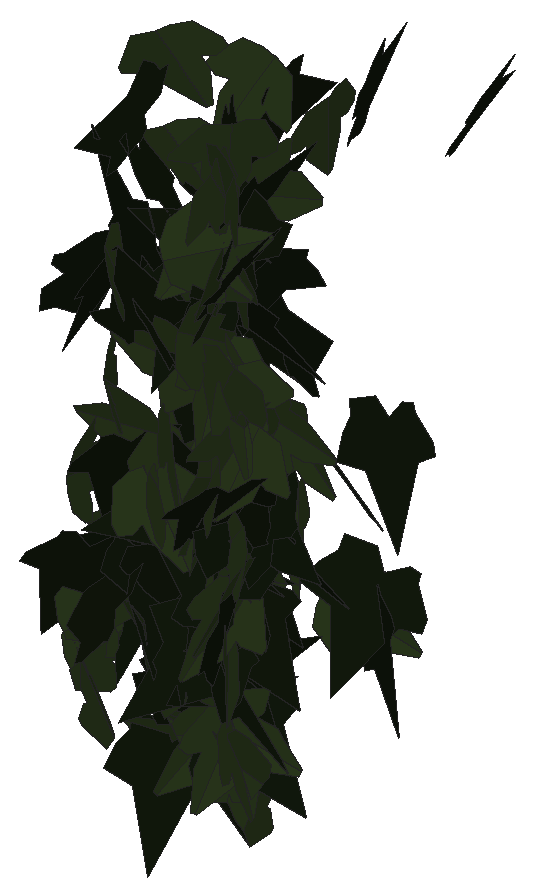
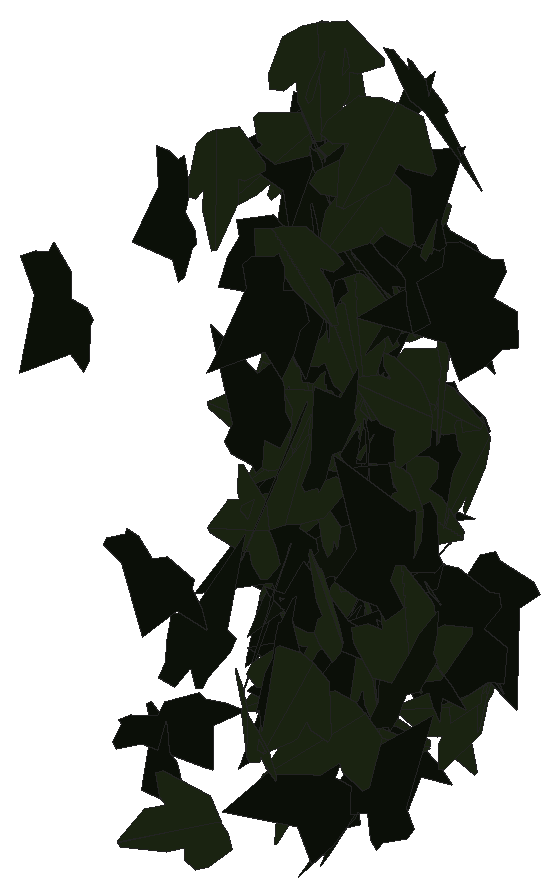
# SketchUp Ruby script. Lengths in inches.
U = 1.inch
M = Sketchup.active_model
def pt(a) = Geom::Point3d.new(a.map { |v| v * U })
def face(e, loops, mat)
  f = e.add_face(loops[0].map { |a| pt(a) })
  loops[1..].each { |l| e.add_face(l.map { |a| pt(a) }).erase! }
  f.material = f.back_material = mat if mat
  f
end
# faces: each face lists its corners as indices into pts; further lists are holes
def faces(e, pts, list, mat = nil) = list.each { |f| face(e, (f[0].is_a?(Array) ? f : [f]).map { |l| l.map { |i| pts[i] } }, mat) }
# xy, xz, yz: faces in a plane at the given z, y or x. An outline is a flat list of corners, or four numbers for a rectangle; further outlines are holes
def ring(l) = l.size == 4 ? [[l[0], l[1]], [l[2], l[1]], [l[2], l[3]], [l[0], l[3]]] : l.each_slice(2).to_a
def flat(e, list, mat, &to3) = list.each { |f| face(e, (f[0].is_a?(Array) ? f : [f]).map { |l| ring(l).map { |u, v| to3.(u, v) } }, mat) }
def xy(e, z, list, mat = nil) = flat(e, list, mat) { |x, y| [x, y, z] }
def xz(e, y, list, mat = nil) = flat(e, list, mat) { |x, z| [x, y, z] }
def yz(e, x, list, mat = nil) = flat(e, list, mat) { |y, z| [x, y, z] }
def lines(e, pts, list) = list.each { |a, b| e.add_line(pt(pts[a]), pt(pts[b])) }
# prism: a flat outline (further loops are holes) pulled along v
def prism(e, loops, v, mat = nil)
  f = face(e, loops, mat); d = Geom::Vector3d.new(v.map { |x| x * U })
  f.pushpull(f.normal.samedirection?(d) ? d.length : -d.length)
end
def box(e, o, s, mat = nil) = prism(e, [[o, [o[0] + s[0], o[1], o[2]], [o[0] + s[0], o[1] + s[1], o[2]], [o[0], o[1] + s[1], o[2]]]], [0, 0, s[2]], mat)
def at(x, y, z, deg = 0) = Geom::Transformation.translation(pt([x, y, z])) * Geom::Transformation.rotation(ORIGIN, Z_AXIS, deg.degrees)
def axes(o, x, y, z) = Geom::Transformation.new([*x, 0, *y, 0, *z, 0, *pt(o).to_a, 1])
def part(name) = M.definitions.add(name)
# library, detail: a bought-in or finely detailed component or shape, given as its bounding box
def library(name, o, s) = part(name).tap { |d| box(d.entities, o, s) }
def detail(e, o, s) = box(e.add_group.entities, o, s)
def put(e, d, t, mat = nil) = e.add_instance(d, t).tap { |i| i.material = mat if mat }
def group(e, t, mat = nil) = e.add_group.tap { |g| g.transformation = t; g.material = mat if mat }.entities
root = M.entities
M.materials.add("efeu1").color = [18, 25, 13]
M.materials.add("efeu2").color = [43, 57, 29]
c1 = part("ivyleaf_9")
p = [[1.54,2.16,1.25],[1.36,2.04,1.19],[-0.21,0.99,0.68],[-0.71,1.11,0.82],[-0.85,0.86,0.67],[-0.8,0.17,0.21],
  [-0.9,-0.01,0.1],[-0.67,-0.16,-0.02],[-0.08,-0.08,-0.05],[-0.03,-0.6,-0.4],[0.65,-0.88,-0.66],[0.83,-0.6,-0.49],
  [1.29,-0.42,-0.43],[1.8125,-0.07,-0.26],[1.21,0.44,0.15]]
faces(c1.entities,p,[[0,1,2,3,4,5,6,7,8,9,10,11,12,13,14]],"efeu1")
c2 = part("ivyleaf_10")
p = [[0,0.5,-0.03],[-0.0625,2.02,-0.43],[-0.19,2.01,-0.46],[-0.54,1.05,-0.29],[-0.52,0.625,-0.18],[-0.83,0.76,-0.28],
  [-1.16,0.64,-0.33],[-1.15,0.33,-0.24],[-0.77,-0.39,0.02],[-0.3,-0.51,0.16],[0.04,-0.48,0.23],[-0.02,2.01,-0.4375],
  [-0.06,2.01,-0.43],[0.04,-0.49,0.23],[0.67,-0.49,0.14],[1.38,0.36,-0.2],[1.375,0.51,-0.24],[0.81,0.65,-0.19],
  [0.62,0.59,-0.15],[0.6,1.09,-0.28],[0.5,1.23,-0.31]]
faces(c2.entities,p,[[0,1,2,3,4,5,6,7,8,9,10],[11,12,0,13,14,15,16,17,18,19,20]],"efeu2")
put(root,c1,axes([43.95,223.39,216.41],[0.08956,-0.30922,0.38258],[0.18004,-0.34128,-0.31799],[0.45778,0.19471,0.05022]))
put(root,c2,axes([44.24,222.97,216.52],[-0.36083,-0.34597,0.01044],[0.01621,-0.00184,0.49973],[-0.34575,0.36097,0.01254]))
put(root,c1,axes([44.42,221.74,216.83],[0.11394,0.33343,-0.35474],[-0.11745,-0.33474,-0.35236],[-0.47246,0.16363,0.00204]))
put(root,c2,axes([44.09,224.26,216.3125],[-0.31231,-0.10129,-0.3771],[0.37075,0.07456,-0.32708],[0.12249,-0.48392,0.02854]))
put(root,c2,axes([44.33,224.72,216.98],[-0.46824,0.06808,-0.16162],[0.15837,-0.03375,-0.47305],[-0.07532,-0.49419,0.01004]))
put(root,c1,axes([44.22,221.66,220.34],[0.04575,0.29571,-0.40057],[0.03546,0.39931,0.29883],[0.49664,-0.05575,0.01557]))
put(root,c2,axes([44.29,221.84,215.41],[0.05774,0.1204,-0.48184],[0.22281,0.42725,0.13346],[0.44387,-0.23013,-0.00431]))
put(root,c2,axes([44.25,221.83,215.86],[0.09592,0.11629,-0.47674],[0.3131,0.35952,0.15069],[0.37784,-0.32745,-0.00385]))
put(root,c1,axes([44.11,221.94,216.47],[0.16385,0.18519,-0.43458],[0.29229,0.3216,0.24726],[0.3711,-0.33508,-0.00287]))
put(root,c1,axes([44.53,222.65,216.38],[-0.41427,-0.07728,-0.26909],[0.2623,0.06092,-0.4213],[0.0979,-0.49022,-0.00993]))
put(root,c2,axes([44.68,221.26,218.1],[-0.03233,0.14031,0.47882],[-0.24713,0.41233,-0.13751],[-0.43345,-0.24556,0.04269]))
put(root,c1,axes([44.72,223.02,214.55],[0.21831,-0.23563,0.38317],[-0.26691,0.27497,0.32117],[-0.36207,-0.34478,-0.00573]))
put(root,c2,axes([44.83,221.46,214.94],[-0.25641,0.20819,-0.37538],[-0.28386,0.24576,0.33019],[0.322,0.38244,-0.00784]))
put(root,c2,axes([44.24,222.9,219.52],[-0.06761,0.04814,-0.49306],[0.4406,-0.22166,-0.08206],[-0.22649,-0.44559,-0.01244]))
put(root,c1,axes([44.78,221.84,220.7],[-0.21326,0.35811,-0.27618],[0.13344,-0.24192,-0.41673],[-0.4321,-0.25145,0.00761]))
put(root,c2,axes([44.59,223.84,217.18],[0.30463,-0.39277,0.05415],[-0.02943,0.0457,0.49704],[-0.39539,-0.30601,0.00472]))
put(root,c2,axes([44.61,222.92,222.875],[-0.40226,-0.22618,-0.19243],[0.16184,0.10468,-0.46136],[0.24899,-0.43346,-0.011]))
put(root,c1,axes([45.02,221.42,216.43],[-0.28644,0.35543,0.20401],[-0.1375,0.15113,-0.45635],[-0.38607,-0.31754,0.01116]))
put(root,c1,axes([44.49,222.68,217.41],[0.22441,0.43966,0.07963],[-0.04676,-0.06551,0.49348],[0.44436,-0.22893,0.01172]))
put(root,c2,axes([44.81,224.32,221.95],[0.45297,-0.0278,-0.20986],[-0.20981,0.00712,-0.4538],[0.02821,0.49918,-0.00521]))
put(root,c2,axes([44.95,221.48,219.3],[-0.16714,0.19657,0.42828],[-0.32378,0.28226,-0.25591],[-0.34238,-0.36289,0.03294]))
put(root,c2,axes([45.09,221.92,217.73],[0.0322,0.02613,-0.49828],[-0.43655,0.24328,-0.01545],[0.24164,0.43604,0.03848]))
put(root,c1,axes([44.84,224.41,221.39],[-0.05763,0.17094,-0.46633],[-0.27081,0.38271,0.17376],[0.41634,0.2726,0.04847]))
put(root,c1,axes([44.57,223.87,219.33],[0.10653,-0.27817,0.40159],[0.13982,-0.37647,-0.29786],[0.46808,0.17576,-0.00243]))
put(root,c1,axes([44.71,224.67,217.1],[0.02397,-0.02602,-0.49875],[0.41184,-0.28143,0.03448],[-0.28252,-0.41246,0.00794]))
put(root,c1,axes([45.23,221.67,222.72],[-0.34868,0.34574,0.09426],[-0.06885,0.06444,-0.49103],[-0.35168,-0.35541,0.00267]))
put(root,c2,axes([45,221.49,220.85],[-0.23258,0.38229,0.22308],[-0.13713,0.17737,-0.44692],[-0.42084,-0.26907,0.02234]))
put(root,c2,axes([44.73,222.33,217.85],[-0.21031,0.20279,-0.40577],[0.27544,-0.29827,-0.29183],[-0.36042,-0.34628,0.01374]))
put(root,c2,axes([45.39,221.52,218.78],[0.0693,0.05687,-0.4919],[-0.47808,0.13707,-0.05151],[0.12899,0.47747,0.07337]))
put(root,c1,axes([45.27,221.58,221.08],[0.10863,-0.16713,0.45855],[-0.24115,0.39004,0.19929],[-0.42432,-0.26446,0.00414]))
put(root,c1,axes([44.82,223.75,221.53],[-0.10787,-0.0159,-0.48797],[0.47869,-0.10172,-0.10251],[-0.09601,-0.48928,0.03717]))
put(root,c1,axes([45.22,221.5,218.57],[0.08551,0.42675,-0.24611],[-0.04554,-0.24187,-0.43523],[-0.49052,0.09685,-0.0025]))
put(root,c2,axes([44.98,222.66,221.87],[-0.4261,-0.10824,-0.23817],[0.23683,0.03382,-0.43906],[0.11115,-0.48697,0.02245]))
put(root,c1,axes([45.14,223.79,219.3],[0.29864,-0.16829,-0.364],[-0.29921,0.20867,-0.34196],[0.26701,0.42206,0.02392]))
put(root,c1,axes([44.97,222.11,216.67],[0.08109,-0.46755,0.15755],[0.04375,-0.15222,-0.47425],[0.49144,0.0907,0.01622]))
put(root,c2,axes([44.95,224.74,216.25],[0.33771,-0.16855,0.32794],[0.29063,-0.15199,-0.37741],[0.22691,0.44552,-0.00468]))
put(root,c1,axes([45.19,223.11,214.77],[-0.01649,0.30684,-0.39443],[-0.11605,0.3815,0.30164],[0.48607,0.1015,0.05864]))
put(root,c2,axes([45.1,221.76,216.02],[-0.31919,0.09275,0.37351],[0.32294,-0.19941,0.32549],[0.20934,0.44903,0.0674]))
put(root,c1,axes([45.08,222.77,214.35],[0.312,-0.38168,-0.08354],[-0.05253,0.06496,-0.49297],[0.38717,0.31639,0.00043]))
put(root,c1,axes([45.4375,222.92,216.43],[-0.46865,0.1147,0.13118],[0.12689,-0.03334,0.48248],[0.11943,0.48552,0.00214]))
put(root,c2,axes([45.65,221.99,215.73],[-0.2024,0.12782,0.43897],[-0.39673,0.1895,-0.2381],[-0.22724,-0.44469,0.02471]))
put(root,c1,axes([45.4,221.73,219.98],[0.39082,0.00991,0.31171],[-0.31178,0.0002,0.39089],[0.00762,-0.4999,0.00634]))
put(root,c1,axes([45.74,222.28,217.61],[-0.34452,-0.10277,0.34748],[-0.33537,-0.09114,-0.35947],[0.13722,-0.48076,-0.00613]))
put(root,c2,axes([45.84,221.6875,219.72],[-0.0287,0.03654,-0.49784],[-0.49175,0.08362,0.03449],[0.08578,0.4916,0.03114]))
put(root,c1,axes([45.21,221.74,222.16],[0.37501,-0.32946,-0.0288],[-0.02157,0.01908,-0.49917],[0.33001,0.37563,0.0001]))
put(root,c1,axes([45.29,221.6875,220.18],[0.43221,-0.20515,-0.14528],[-0.1297,0.06553,-0.47842],[0.21533,0.45124,0.00343]))
put(root,c2,axes([45.86,221.93,214.625],[-0.04687,0.06085,-0.49407],[-0.49089,0.07671,0.05602],[0.08262,0.49032,0.05255]))
put(root,c1,axes([45.76,221.88,218.2],[0.06133,0.01034,-0.49612],[-0.48755,0.0943,-0.0583],[0.09237,0.49092,0.02165]))
put(root,c1,axes([45.51,221.84,214.64],[-0.38908,-0.18308,-0.25515],[0.22968,0.11113,-0.42999],[0.21415,-0.45181,-0.00238]))
put(root,c2,axes([45.59,221.57,218.12],[-0.12618,0.41556,0.24776],[-0.09726,0.22903,-0.43369],[-0.47394,-0.15764,0.02304]))
put(root,c2,axes([45.67,223.15,217.92],[0.2006,0.45742,0.02291],[-0.01516,-0.01836,0.49943],[0.45775,-0.20106,0.0065]))
put(root,c2,axes([45.54,221.78,215.49],[0.3498,-0.35584,-0.03197],[0.03042,-0.01491,0.49885],[-0.35597,-0.35094,0.01121]))
put(root,c2,axes([45.61,221.77,218.85],[-0.08912,0.47909,-0.11194],[0.02161,-0.10984,-0.48731],[-0.49152,-0.0917,-0.00113]))
put(root,c1,axes([45.76,222.15,220.65],[-0.45514,-0.13017,-0.16095],[0.15423,0.04603,-0.47339],[0.13806,-0.48056,-0.00175]))
put(root,c1,axes([45.4,221.79,217.21],[0.04248,0.08592,-0.49073],[0.22287,0.4372,0.09584],[0.44556,-0.22688,-0.00116]))
put(root,c2,axes([45.73,221.95,219.97],[0.47583,0.1375,-0.06842],[-0.12064,0.19676,-0.44354],[-0.09505,0.43861,0.22043]))
put(root,c1,axes([45.7,224.8125,216.77],[0.34973,-0.34949,0.07449],[-0.0505,0.05484,0.49441],[-0.35375,-0.35334,0.00306]))
put(root,c2,axes([45.49,221.51,218.09],[0.3848,0.20368,0.24585],[0.20792,0.1323,-0.43504],[-0.24227,0.43705,0.01712]))
put(root,c2,axes([45.4,225.05,215],[0.15532,0.10871,0.46266],[0.39578,0.23989,-0.18923],[-0.26312,0.42501,-0.01153]))
put(root,c2,axes([45.89,222.08,219.57],[0.43171,0.12565,-0.21872],[-0.24936,0.14732,-0.40757],[-0.03798,0.46099,0.18986]))
put(root,c1,axes([46.03,221.95,220.73],[-0.43248,0.24746,-0.04153],[0.03339,-0.02525,-0.49824],[-0.24868,-0.43374,0.00532]))
put(root,c1,axes([46.11,221.97,218.81],[0.13011,-0.06997,0.47768],[-0.4333,0.20123,0.1475],[-0.21289,-0.45234,-0.00827]))
put(root,c1,axes([45.85,222.13,221.53],[0.42166,0.12539,-0.23766],[-0.26707,0.14685,-0.39637],[-0.0296,0.46121,0.19082]))
put(root,c2,axes([45.89,222.18,217.55],[0.117,-0.47774,0.08989],[0.02513,-0.08639,-0.49184],[0.48547,0.11961,0.0038]))
put(root,c1,axes([45.87,222.55,215.59],[-0.11988,-0.24896,0.41671],[-0.10508,-0.40574,-0.27264],[0.47391,-0.15294,0.04495]))
put(root,c1,axes([45.57,221.75,215.3125],[0.20069,0.01142,0.45781],[0.44597,0.10872,-0.19821],[-0.10407,0.4879,0.03346]))
put(root,c2,axes([46.12,221.92,217.375],[-0.46581,-0.05211,0.17408],[-0.17237,-0.02485,-0.46869],[0.0575,-0.49666,0.00518]))
put(root,c1,axes([45.66,223.6875,219.07],[0.01758,-0.04727,0.49745],[0.29108,-0.40362,-0.04864],[0.40616,0.29131,0.01332]))
put(root,c1,axes([46.16,221.95,216.15],[-0.35903,-0.28059,0.20583],[-0.16387,-0.12457,-0.45566],[0.30698,-0.39466,-0.00251]))
put(root,c1,axes([45.92,222.16,217.125],[0.45736,0.13702,-0.14848],[-0.19396,0.19484,-0.41763],[-0.05659,0.43962,0.23138]))
put(root,c2,axes([46.08,221.85,218.22],[0.03618,0.02473,-0.49808],[-0.03761,0.4981,0.022],[0.49727,0.03587,0.0379]))
put(root,c2,axes([46.13,221.87,221.45],[0.3792,0.1705,-0.27773],[-0.25775,-0.10384,-0.41567],[-0.19943,0.45842,0.00914]))
put(root,c1,axes([46.38,221.84,216.91],[-0.07722,0.1549,0.46909],[-0.45431,0.1642,-0.12901],[-0.19402,-0.44614,0.11539]))
put(root,c1,axes([46.14,222.57,220.76],[0.19583,0.38751,-0.24797],[-0.11994,-0.21718,-0.43411],[-0.44415,0.2295,0.00789]))
put(root,c2,axes([45.99,222.05,215.95],[0.05669,0.2304,-0.44012],[0.10608,0.42714,0.23727],[0.48532,-0.12027,-0.00045]))
put(root,c2,axes([45.66,223.72,217.92],[0.17131,-0.06074,0.46579],[0.46771,-0.02394,-0.17514],[0.04357,0.49572,0.04862]))
put(root,c1,axes([46.14,221.99,217.55],[0.34596,-0.09306,0.34879],[-0.32275,0.13667,0.35659],[-0.1617,-0.47187,0.03449]))
put(root,c2,axes([46.15,221.9,215.1],[0.16474,0.26573,-0.39019],[-0.20689,-0.33083,-0.31265],[-0.42433,0.26447,0.00095]))
put(root,c1,axes([46.17,224.41,221.91],[0.02411,0.15615,0.47438],[0.07829,0.46788,-0.15798],[-0.49324,0.0819,-0.00189]))
put(root,c2,axes([46.22,221.61,218.49],[0.3537,-0.29177,-0.19942],[-0.14065,0.14261,-0.45813],[0.32421,0.38017,0.0188]))
put(root,c2,axes([45.78,221.79,221.08],[-0.11615,-0.00503,-0.4863],[0.46353,-0.15241,-0.10914],[-0.14713,-0.47618,0.04007]))
put(root,c2,axes([46.1875,221.41,220.33],[0.01124,0.24269,0.437],[-0.13682,0.42192,-0.23079],[-0.48078,-0.1144,0.0759]))
put(root,c2,axes([46.49,221.91,214.63],[-0.26746,-0.00833,-0.42237],[-0.4205,-0.04284,0.26711],[-0.04064,0.49809,0.01591]))
put(root,c1,axes([46.23,221.98,221.49],[-0.38019,0.18184,-0.26906],[0.24444,-0.11249,-0.42142],[-0.21379,-0.45198,-0.00337]))
put(root,c2,axes([46.15,221.97,219.8],[0.19888,0.42658,-0.16876],[-0.08062,-0.14857,-0.47056],[-0.45161,0.21438,0.00969]))
put(root,c2,axes([46.24,221.96,221.16],[-0.42143,0.26371,0.05342],[-0.04405,0.03032,-0.49713],[-0.26544,-0.42372,-0.00232]))
put(root,c1,axes([46.52,221.95,221.21],[-0.08059,0.00355,0.49345],[-0.48872,-0.06972,-0.07931],[0.06825,-0.4951,0.0147]))
put(root,c2,axes([46.18,222.02,216.99],[0.02312,0.21108,0.45267],[-0.05494,0.45148,-0.20772],[-0.49643,-0.04013,0.04407]))
put(root,c1,axes([46.22,222.57,216.82],[0.257,-0.17095,-0.39335],[-0.33132,0.21206,-0.30863],[0.27236,0.41929,-0.00428]))
put(root,c2,axes([46.2,221.61,218.48],[-0.05295,-0.23742,-0.43684],[0.09485,0.42642,-0.24325],[0.48806,-0.10863,-0.00012]))
put(root,c2,axes([46.27,223.67,222.26],[-0.03362,-0.48606,-0.1123],[0.02125,0.11106,-0.48705],[0.49842,-0.03752,0.01319]))
put(root,c2,axes([46.41,221.8,217.6875],[0.33819,-0.20505,-0.30591],[-0.2281,0.20945,-0.39256],[0.28913,0.40507,0.04813]))
put(root,c1,axes([45.97,222.3125,220.34],[0.4945,-0.041,0.06153],[0.06068,-0.01273,-0.49614],[0.04225,0.49815,-0.00761]))
put(root,c1,axes([46.26,224.67,215.84],[-0.29416,-0.40418,-0.01026],[0.00596,0.00835,-0.49989],[0.40427,-0.29422,-0.00009]))
put(root,c2,axes([46.36,221.86,222.74],[-0.30303,-0.39766,0.00638],[-0.00309,-0.00567,-0.49996],[0.3977,-0.30305,0.00097]))
put(root,c2,axes([46.1,222.05,218.32],[0.14223,0.21718,0.42732],[0.15224,0.40219,-0.25508],[-0.45453,0.20267,0.04828]))
put(root,c2,axes([46.32,221.92,215.11],[0.25265,0.37079,-0.22064],[-0.14125,-0.17051,-0.4483],[-0.4077,0.28886,0.01859]))
put(root,c2,axes([46.33,222.21,213.96],[0.01752,0.22469,-0.44633],[0.01587,0.44613,0.22521],[0.49944,-0.02205,0.0085]))
put(root,c1,axes([46.01,222.7,217.35],[0.4841,-0.10126,0.07345],[0.07146,-0.01709,-0.49457],[0.10267,0.48934,-0.00207]))
put(root,c1,axes([46.32,221.96,221.49],[-0.05446,0.41577,-0.27233],[-0.1733,0.24089,0.40242],[0.46583,0.13822,0.11787]))
put(root,c2,axes([46.57,221.61,219.84],[-0.43268,-0.00419,0.25054],[-0.24978,-0.0326,-0.43191],[0.01995,-0.49892,0.02612]))
put(root,c1,axes([46.57,221.53,218.38],[-0.0506,0.42845,-0.25273],[-0.0844,-0.25775,-0.42005],[-0.49022,0.00016,0.09841]))
put(root,c2,axes([46.01,221.49,221.3],[0.12888,0.0308,-0.48212],[0.4652,0.12668,0.13245],[0.1303,-0.48271,0.004]))
put(root,c1,axes([46.21,222.11,216.5625],[-0.02342,-0.29235,-0.40495],[0.01949,0.40455,-0.29319],[0.49907,-0.02952,-0.00756]))
put(root,c2,axes([46.42,221.55,221.32],[0.17407,-0.43167,-0.18265],[-0.02957,0.18434,-0.46384],[0.46779,0.17228,0.03864]))
put(root,c1,axes([46.72,222.12,217.65],[-0.40878,0.03966,-0.28518],[-0.28392,0.02679,0.4107],[0.04786,0.4977,0.00062]))
put(root,c2,axes([46.34,222.375,221.76],[-0.0098,0.18146,0.46581],[-0.02665,0.46505,-0.18172],[-0.49919,-0.02839,0.00056]))
put(root,c1,axes([46.2,222.0625,215.87],[0.30138,-0.35547,-0.18114],[-0.10985,0.1443,-0.46595],[0.38354,0.32066,0.00888]))
put(root,c1,axes([46.2,222.07,215.18],[0.0345,-0.30093,-0.39781],[0.04287,0.39907,-0.29817],[0.49696,-0.01353,0.05334]))
put(root,c2,axes([46.44,221.79,216.82],[0.15077,0.32443,-0.3493],[-0.15961,-0.31086,-0.35762],[-0.44921,0.21934,0.00983]))
put(root,c1,axes([46.57,221.41,216.8],[-0.06037,0.10703,-0.48467],[-0.36434,0.322,0.11649],[0.33706,0.36723,0.03911]))
put(root,c2,axes([46.48,221.92,219.05],[-0.13374,-0.48148,-0.017],[0.00459,0.01637,-0.49971],[0.48176,-0.13382,0.00004]))
put(root,c1,axes([46.28,224.78,217.77],[-0.30763,-0.13136,-0.37163],[0.34252,0.14419,-0.3345],[0.19505,-0.46039,0.00127]))
put(root,c2,axes([46.33,221.93,216.32],[-0.12443,0.39434,-0.28109],[0.06155,-0.27499,-0.41303],[-0.48034,-0.13739,0.01989]))
put(root,c2,axes([46.375,221.95,215.06],[-0.06513,0.49564,0.01014],[-0.00393,0.00971,-0.49989],[-0.49572,-0.06519,0.00263]))
put(root,c2,axes([46.4,221.52,222.31],[0.03383,-0.42671,-0.2584],[0.10244,0.25942,-0.41498],[0.48822,-0.02486,0.10498]))
put(root,c2,axes([46.53,221.92,217.08],[-0.11115,0.33205,-0.35692],[-0.16057,-0.37059,-0.29476],[-0.46029,0.04909,0.18901]))
put(root,c1,axes([46.21,224.61,215.38],[-0.1191,0.00591,-0.48557],[0.48554,-0.00681,-0.11917],[-0.00802,-0.49992,-0.00412]))
put(root,c1,axes([46.31,221.98,217.99],[0.0318,-0.20128,-0.45659],[0.01124,0.45769,-0.20098],[0.49886,0.00252,0.03364]))
put(root,c1,axes([46.55,221.49,221.07],[0.09659,0.38495,0.30411],[0.03965,0.30281,-0.3959],[-0.48898,0.10059,0.02796]))
put(root,c1,axes([46.61,225.8,221.3],[0.052,0.32405,0.37721],[0.03927,0.37541,-0.32791],[-0.49574,0.06373,0.01359]))
put(root,c2,axes([46.64,221.43,222.46],[0.3313,-0.19621,-0.31897],[-0.17028,0.30037,-0.36164],[0.33353,0.34825,0.13221]))
put(root,c2,axes([46.21,221.875,215.14],[0.16374,0.15784,0.44528],[0.32858,0.30056,-0.22737],[-0.33945,0.36708,-0.0053]))
put(root,c2,axes([46.14,222.85,218.59],[0.02068,-0.03046,0.49864],[0.49708,0.05101,-0.0175],[-0.04981,0.49646,0.03239]))
put(root,c2,axes([46.47,221.92,219.53],[0.07694,0.49313,-0.03007],[-0.00782,-0.02921,-0.49908],[-0.49398,0.07727,0.00322]))
put(root,c2,axes([46.59,221.87,218.86],[0.4758,0.05792,-0.14234],[-0.14365,0.00309,-0.47891],[-0.05459,0.49662,0.01958]))
